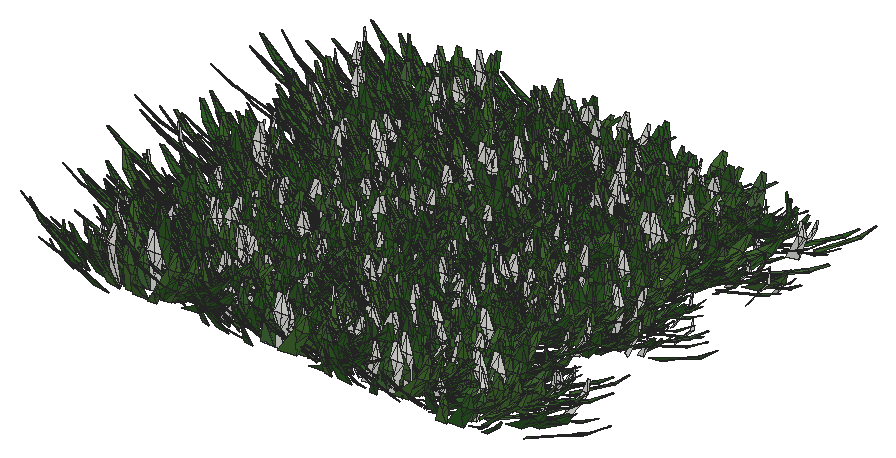
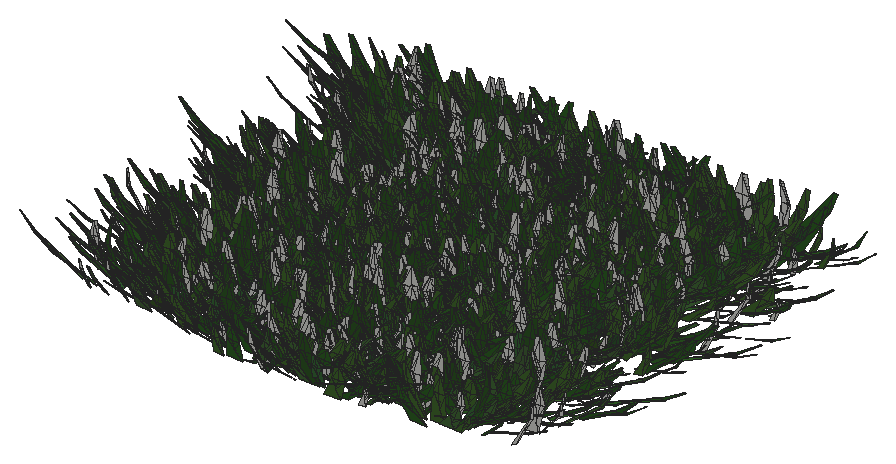
# SketchUp Ruby script. Lengths in inches.
U = 1.inch
M = Sketchup.active_model
def pt(a) = Geom::Point3d.new(a.map { |v| v * U })
def face(e, loops, mat)
  f = e.add_face(loops[0].map { |a| pt(a) })
  loops[1..].each { |l| e.add_face(l.map { |a| pt(a) }).erase! }
  f.material = f.back_material = mat if mat
  f
end
# faces: each face lists its corners as indices into pts; further lists are holes
def faces(e, pts, list, mat = nil) = list.each { |f| face(e, (f[0].is_a?(Array) ? f : [f]).map { |l| l.map { |i| pts[i] } }, mat) }
# xy, xz, yz: faces in a plane at the given z, y or x. An outline is a flat list of corners, or four numbers for a rectangle; further outlines are holes
def ring(l) = l.size == 4 ? [[l[0], l[1]], [l[2], l[1]], [l[2], l[3]], [l[0], l[3]]] : l.each_slice(2).to_a
def flat(e, list, mat, &to3) = list.each { |f| face(e, (f[0].is_a?(Array) ? f : [f]).map { |l| ring(l).map { |u, v| to3.(u, v) } }, mat) }
def xy(e, z, list, mat = nil) = flat(e, list, mat) { |x, y| [x, y, z] }
def xz(e, y, list, mat = nil) = flat(e, list, mat) { |x, z| [x, y, z] }
def yz(e, x, list, mat = nil) = flat(e, list, mat) { |y, z| [x, y, z] }
def lines(e, pts, list) = list.each { |a, b| e.add_line(pt(pts[a]), pt(pts[b])) }
# prism: a flat outline (further loops are holes) pulled along v
def prism(e, loops, v, mat = nil)
  f = face(e, loops, mat); d = Geom::Vector3d.new(v.map { |x| x * U })
  f.pushpull(f.normal.samedirection?(d) ? d.length : -d.length)
end
def box(e, o, s, mat = nil) = prism(e, [[o, [o[0] + s[0], o[1], o[2]], [o[0] + s[0], o[1] + s[1], o[2]], [o[0], o[1] + s[1], o[2]]]], [0, 0, s[2]], mat)
def at(x, y, z, deg = 0) = Geom::Transformation.translation(pt([x, y, z])) * Geom::Transformation.rotation(ORIGIN, Z_AXIS, deg.degrees)
def axes(o, x, y, z) = Geom::Transformation.new([*x, 0, *y, 0, *z, 0, *pt(o).to_a, 1])
def part(name) = M.definitions.add(name)
# library, detail: a bought-in or finely detailed component or shape, given as its bounding box
def library(name, o, s) = part(name).tap { |d| box(d.entities, o, s) }
def detail(e, o, s) = box(e.add_group.entities, o, s)
def put(e, d, t, mat = nil) = e.add_instance(d, t).tap { |i| i.material = mat if mat }
def group(e, t, mat = nil) = e.add_group.tap { |g| g.transformation = t; g.material = mat if mat }.entities
root = M.entities
M.materials.add("Material10").color = [48, 100, 38]
M.materials.add("Material3").color = [68, 110, 58]
M.materials.add("Material4").color = [48, 90, 38]
M.materials.add("Material5").color = [68, 110, 48]
M.materials.add("Material6").color = [48, 90, 48]
M.materials.add("Material7").color = [58, 110, 58]
M.materials.add("Material8").color = [58, 90, 38]
M.materials.add("Material9").color = [68, 100, 58]
c1 = part("grass00")
p = [[-0.6875,0.15,0],[-0.56,0.08,5.52],[-0.04,0.03,2.76],[0.48,-0.02,0],[0.35,-0.02,5.52],[-0.1,-0.14,5.52],
  [-0.12,0.65,8.37],[-0.42,0.65,8.37]]
faces(c1.entities,p,[[0,1,2,3],[3,2,4],[1,5,2],[5,4,2],[1,6,5],[4,5,6],[7,6,1]])
c2 = part("Group16\#1")
put(c2.entities,c1,axes([1.44,-0.61,-0.01],[0.05352,0.12609,0],[-0.10704,0.04543,0.07239],[0.06664,-0.02828,0.11628]),"Material6")
put(c2.entities,c1,axes([0.76,-0.15,-0.01],[0.04676,0.24062,0],[-0.23162,0.04501,0.06642],[0.0652,-0.01267,0.23595]),"Material3")
put(c2.entities,c1,axes([0.79,0.01,-0.01],[-0.00606,0.34651,0],[-0.34381,-0.00602,0.0432],[0.04319,0.00076,0.34386]))
put(c2.entities,c1,axes([1,0.23,-0.01],[-0.07192,0.31144,0],[-0.28722,-0.06632,0.1236],[0.12043,0.02781,0.29478]),"Material5")
put(c2.entities,c1,axes([1.66,0.77,-0.01],[-0.13828,0.29651,0],[-0.21551,-0.1005,0.22471],[0.20365,0.09498,0.23779]),"Material10")
put(c2.entities,c1,axes([0.6875,0.52,-0.01],[-0.18126,0.24051,0],[-0.22746,-0.17142,0.09788],[0.07817,0.05891,0.28481]),"Material5")
put(c2.entities,c1,axes([0.68,0.78,-0.01],[-0.215,0.18688,0],[-0.12385,-0.14248,0.21334],[0.13995,0.16101,0.18878]),"Material3")
put(c2.entities,c1,axes([0.56,1,-0.01],[-0.13756,0.07624,0],[-0.06159,-0.11112,0.0927],[0.04494,0.08108,0.12705]),"Material5")
put(c2.entities,c1,axes([0.2,0.64,-0.01],[-0.23729,0.07254,0],[-0.05711,-0.18681,0.153],[0.04473,0.14632,0.19535]),"Material10")
put(c2.entities,c1,axes([0.0625,0.72,-0.01],[-0.28874,0.02525,0],[-0.02179,-0.24916,0.14647],[0.01276,0.14591,0.25012]),"Material3")
put(c2.entities,c1,axes([-0.08,0.62,-0.01],[-0.34089,-0.04187,0],[0.03255,-0.26504,0.216],[-0.02633,0.21439,0.26703]),"Material10")
put(c2.entities,c1,axes([-0.34,0.98,-0.01],[-0.14314,-0.0493,0],[0.04397,-0.12769,0.06843],[-0.02228,0.0647,0.13505]),"Material10")
put(c2.entities,c1,axes([-0.87,1.45,-0.01],[-0.23488,-0.14114,0],[0.13761,-0.22901,0.06087],[-0.03135,0.05217,0.26717]))
put(c2.entities,c1,axes([-0.72,0.77,-0.01],[-0.14208,-0.13251,0],[0.07209,-0.0773,0.16301],[-0.11118,0.11922,0.1057]),"Material10")
put(c2.entities,c1,axes([-0.62,0.43,-0.01],[-0.14845,-0.21203,0],[0.18654,-0.13061,0.12304],[-0.10079,0.07057,0.22772]),"Material3")
put(c2.entities,c1,axes([-0.68,0.29,-0.01],[-0.13639,-0.32136,0],[0.31723,-0.13464,0.05579],[-0.05136,0.0218,0.34462]),"Material4")
put(c2.entities,c1,axes([-0.64,0.125,-0.01],[-0.0458,-0.23569,0],[0.22124,-0.043,0.08276],[-0.08124,0.01579,0.22538]),"Material7")
put(c2.entities,c1,axes([-1.6,-0.03,-0.01],[0.00576,-0.32897,0],[0.27526,0.00482,0.18018],[-0.18015,-0.00315,0.2753]),"Material5")
put(c2.entities,c1,axes([-1.36,-0.31,-0.01],[0.05718,-0.24765,0],[0.18172,0.04196,0.17267],[-0.16825,-0.03885,0.1865]),"Material10")
put(c2.entities,c1,axes([-1.54,-0.72,-0.01],[0.06537,-0.14017,0],[0.13555,0.06321,0.03939],[-0.0357,-0.01665,0.14956]))
put(c2.entities,c1,axes([-1.19,-0.9,-0.01],[0.09597,-0.12735,0],[0.11214,0.08451,0.07557],[-0.06035,-0.04548,0.14042]),"Material9")
put(c2.entities,c1,axes([-0.47,-0.54,-0.01],[0.11588,-0.10072,0],[0.0618,0.0711,0.12124],[-0.07953,-0.0915,0.0942]))
put(c2.entities,c1,axes([-0.47,-0.84,-0.01],[0.11927,-0.0661,0],[0.06603,0.11913,0.00646],[-0.00313,-0.00565,0.13621]),"Material5")
put(c2.entities,c1,axes([-0.38,-1.24,-0.01],[0.28037,-0.08571,0],[0.0618,0.20215,0.20315],[-0.05939,-0.19428,0.21139]),"Material9")
put(c2.entities,c1,axes([-0.06,-0.66,-0.01],[0.22719,-0.01987,0],[0.01247,0.14255,0.17758],[-0.01547,-0.17691,0.1431]),"Material8")
put(c2.entities,c1,axes([0.11,-0.89,-0.01],[0.14882,0.01828,0],[-0.01058,0.08611,0.12229],[0.01491,-0.12138,0.08676]),"Material6")
put(c2.entities,c1,axes([0.25,-0.72,-0.01],[0.20481,0.07053,0],[-0.06206,0.18022,0.10291],[0.03351,-0.0973,0.1906]),"Material6")
put(c2.entities,c1,axes([0.85,-1.42,-0.01],[0.16481,0.09904,0],[-0.09472,0.15762,0.05616],[0.02893,-0.04814,0.18389]),"Material5")
put(c2.entities,c1,axes([1.01,-1.09,-0.01],[0.21858,0.20385,0],[-0.17495,0.1876,0.15339],[0.10462,-0.11218,0.25652]),"Material10")
put(c2.entities,c1,axes([1.01,-0.71,-0.01],[0.08733,0.12473,0],[-0.06445,0.04512,0.13037],[0.1068,-0.07477,0.07867]),"Material6")
c3 = part("Group15\#1")
put(c3.entities,c2,at(0,0,0))
c4 = part("3darcstudiotree_grass00\#1")
put(c4.entities,c3,at(0,0,0))
put(root,c4,axes([922.19,902.96,0],[3.02119,-0.73797,0],[3.34783,0.85662,-0.03867],[0.15719,0.04022,1.7417]))
put(root,c4,axes([921.78,912.33,0],[-0.66076,1.04694,0],[-4.20152,-0.16573,-0.0149],[-0.10633,-0.00419,1.9212]))
put(root,c4,axes([924.36,916.55,0],[-4.31344,-0.70765,0],[2.03692,-0.77599,-0.04657],[0.20265,-0.0772,1.84036]))
put(root,c4,axes([924.04,895.31,0],[1.44261,-1.06055,0],[4.32057,0.36732,-0.01889],[0.12331,0.01048,1.96679]))
put(root,c4,axes([923.94,921.2,0],[2.7969,-0.77222,0],[3.1053,0.70294,-0.04299],[0.19432,0.04399,1.59659]))
put(root,c4,axes([924.92,894.38,0],[-3.32225,-0.97797,0],[3.38352,-0.71838,-0.05304],[0.28473,-0.06045,1.95407]))
put(root,c4,axes([924.86,922.86,0],[-4.68241,-0.00671,0],[0.02158,-0.94079,-0.00073],[0.00003,-0.00117,1.50826]))
put(root,c4,axes([924.16,924.21,0],[-2.30847,0.97502,0],[-3.8485,-0.56948,-0.03668],[-0.22363,-0.03309,1.98009]))
put(root,c4,axes([924.59,907.05,0],[-3.40463,0.90031,0],[-2.90136,-0.68574,-0.02847],[-0.11642,-0.02752,1.40417]))
put(root,c4,axes([925.07,925.48,0],[-3.76475,0.39529,0],[-1.59865,-0.95161,-0.01995],[-0.04859,-0.02892,1.62326]))
put(root,c4,axes([924.7,900.36,0],[-2.71864,0.85934,0],[-2.93369,-0.58007,-0.01059],[-0.0476,-0.00941,1.33934]))
put(root,c4,axes([925.75,913.93,0],[-4.9722,0.10596,0],[-0.33395,-0.9794,-0.04632],[-0.03038,-0.08909,1.89764]))
put(root,c4,axes([924,927.71,0],[3.97374,0.24333,0],[-1.22585,1.25118,-0.01455],[-0.02127,0.02171,1.97892]))
put(root,c4,axes([926.76,914.61,0],[-4.53093,-0.46907,0],[1.45069,-0.87579,-0.00358],[0.00956,-0.00577,1.65637]))
put(root,c4,axes([925.76,919.37,0],[-1.34638,0.95238,0],[-3.42274,-0.30242,-0.03966],[-0.22852,-0.02019,1.38647]))
put(root,c4,axes([926.29,911.04,0],[-3.83366,0.85497,0],[-2.76672,-0.77537,-0.04505],[-0.16078,-0.04506,1.39266]))
put(root,c4,axes([927.32,917.65,0],[-1.48823,-0.96446,0],[4.19205,-0.40429,-0.03571],[0.22835,-0.02202,1.92492]))
put(root,c4,axes([925.79,931.9375,0],[2.1454,0.98431,0],[-3.66531,0.49931,-0.025],[-0.16769,0.02284,1.99255]))
put(root,c4,axes([927.59,912.1,0],[-4.49935,0.03553,0],[-0.13779,-1.09065,-0.03959],[-0.00757,-0.05991,1.65212]))
put(root,c4,axes([926.65,904.93,0],[3.94822,-0.31947,0],[1.46453,1.13124,-0.01611],[0.0264,0.02039,1.58139]))
put(root,c4,axes([925.95,905.5,0],[3.048,0.98317,0],[-3.94868,0.7651,-0.03267],[-0.16044,0.03109,1.93988]))
put(root,c4,axes([926.13,929.33,0],[1.55836,1.05765,0],[-4.59334,0.423,-0.04046],[-0.19369,0.01784,1.56076]))
put(root,c4,axes([926.24,902.52,0],[0.02941,0.96921,0],[-5.11425,0.0097,-0.03677],[-0.15931,0.0003,1.38481]))
put(root,c4,axes([928.14,896.83,0],[-4.27197,-0.09913,0],[0.4691,-1.26352,-0.06502],[0.02705,-0.07286,1.42798]))
put(root,c4,axes([927.1,908.91,0],[-0.64236,0.88776,0],[-3.75703,-0.1699,-0.01415],[-0.08369,-0.00378,1.43376]))
put(root,c4,axes([928.22,901.49,0],[1.50582,-1.13859,0],[4.62077,0.38195,-0.04027],[0.21526,0.01779,1.71232]))
put(root,c4,axes([928.3125,930,0],[3.80605,-0.38984,0],[1.42887,0.87189,-0.00746],[0.01834,0.01119,1.52751]))
put(root,c4,axes([927.69,898.05,0],[3.10025,0.78829,0],[-3.57532,0.87883,-0.00938],[-0.04176,0.01026,1.95578]))
put(root,c4,axes([930.625,910.42,0],[-1.03913,-0.96879,0],[4.9712,-0.33326,-0.04199],[0.22449,-0.01505,1.7807]))
put(root,c4,axes([931.02,914.85,0],[-2.80799,-0.72862,0],[3.20036,-0.77086,-0.03217],[0.13224,-0.03185,1.58546]))
put(root,c4,axes([930.6875,901.37,0],[-4.63896,0.21302,0],[-0.93332,-1.27031,-0.05609],[-0.06093,-0.08294,1.94158]))
put(root,c4,axes([930.97,908.14,0],[-4.20413,-0.53147,0],[1.63067,-0.8062,-0.0255],[0.09899,-0.04894,1.94297]))
put(root,c4,axes([930.6,927.73,0],[-3.90893,0.68034,0],[-2.78299,-0.99937,-0.02528],[-0.08388,-0.03012,1.76765]))
put(root,c4,axes([930.33,898.82,0],[0.1527,1.05059,0],[-3.86386,0.0351,-0.04285],[-0.32383,0.00294,1.82733]))
put(root,c4,axes([930.53,926.14,0],[3.71157,-0.27079,0],[1.39023,1.19096,-0.04654],[0.05647,0.04838,1.34343]))
put(root,c4,axes([930.24,931.74,0],[3.97715,0.44667,0],[-1.63668,0.9108,-0.04301],[-0.1186,0.066,1.6797]))
put(root,c4,axes([930.86,908.72,0],[3.86502,-0.35215,0],[1.63703,1.12296,-0.06136],[0.12705,0.08716,1.80687]))
put(root,c4,axes([932.39,900.08,0],[-0.56967,-1.02254,0],[3.9547,-0.1377,-0.01078],[0.07697,-0.00268,1.79898]))
put(root,c4,axes([932.79,916.45,0],[-1.46525,-0.90866,0],[3.94836,-0.39793,-0.00075],[0.00398,-0.0004,1.52674]))
put(root,c4,axes([931.21,903.43,0],[4.11417,0.05124,0],[-0.24086,1.20875,-0.00527],[-0.00138,0.00693,1.59512]))
put(root,c4,axes([933.53,930.17,0],[-2.16831,-1.16182,0],[4.23849,-0.49439,-0.01753],[0.08143,-0.0095,1.49864]))
put(root,c4,axes([932.22,921.73,0],[3.83036,-0.81769,0],[2.5645,0.75081,-0.01134],[0.04499,0.01317,1.5074]))
put(root,c4,axes([933.03,897.48,0],[-4.70771,0.35936,0],[-1.47237,-1.20555,-0.03433],[-0.04305,-0.03525,1.35329]))
put(root,c4,axes([932.8,917.68,0],[-3.29867,0.81125,0],[-2.71253,-0.68934,-0.0233],[-0.12397,-0.0315,1.83382]))
put(root,c4,axes([932.52,919.77,0],[-0.78138,1.08578,0],[-4.54266,-0.20432,-0.02584],[-0.11477,-0.00516,1.30174]))
put(root,c4,axes([933.79,923.92,0],[2.17808,-0.78505,0],[4.26827,0.74013,-0.02169],[0.08641,0.01498,1.57389]))
put(root,c4,axes([932.86,904.5,0],[-0.70651,0.89155,0],[-4.48869,-0.22232,-0.03573],[-0.20534,-0.01017,1.67549]))
put(root,c4,axes([934.39,895.2,0],[-3.74457,-0.22418,0],[0.88563,-0.92456,-0.00326],[0.00619,-0.00646,1.93944]))
put(root,c4,axes([932.75,906.34,0],[3.07381,0.68375,0],[-2.58138,0.72529,-0.00943],[-0.03598,0.01011,1.39243]))
put(root,c4,axes([933.5625,911.76,0],[-0.98652,1.16576,0],[-4.8711,-0.25764,-0.05558],[-0.27807,-0.01471,1.59125]))
put(root,c4,axes([934.34,928.53,0],[1.84217,-1.02173,0],[3.32278,0.37443,-0.02223],[0.14494,0.01633,1.62899]))
put(root,c4,axes([934.43,922.28,0],[3.84212,-0.38705,0],[1.37613,0.85378,-0.02314],[0.05053,0.03135,1.34449]))
put(root,c4,axes([933.86,913.49,0],[1.9287,1.10406,0],[-3.72338,0.40653,-0.01938],[-0.11115,0.01214,1.58937]))
put(root,c4,axes([936.25,907.91,0],[-1.7561,-0.89869,0],[3.62331,-0.44251,-0.0349],[0.22933,-0.02801,1.84302]))
put(root,c4,axes([936.89,917.16,0],[-4.2283,-0.0064,0],[0.03055,-1.26138,-0.0591],[0.00173,-0.07136,1.52309]))
put(root,c4,axes([937.11,914.2,0],[-4.7095,-0.098,0],[0.36806,-1.10545,-0.036],[0.02101,-0.06311,1.9513]))
put(root,c4,axes([936.86,925.27,0],[1.82992,-1.20621,0],[3.40004,0.32238,-0.00605],[0.04862,0.00461,1.95327]))
put(root,c4,axes([936.97,933.53,0],[1.45443,-0.84507,0],[4.00274,0.43056,-0.02985],[0.15547,0.01672,1.54439]))
put(root,c4,axes([936.65,922.17,0],[0.91767,-0.96683,0],[3.51247,0.20837,-0.04624],[0.38905,0.02308,1.95114]))
put(root,c4,axes([936.64,928.94,0],[-2.22547,0.97496,0],[-3.23871,-0.46204,-0.04437],[-0.2422,-0.03455,1.46464]))
put(root,c4,axes([936.25,899.97,0],[-1.07117,1.0548,0],[-4.16401,-0.26429,-0.01715],[-0.09038,-0.00574,1.46021]))
put(root,c4,axes([937.97,918,0],[-0.7412,-1.17343,0],[4.56586,-0.18025,-0.01303],[0.08774,-0.00346,1.96953]))
put(root,c4,axes([937.62,894.28,0],[1.34034,-1.07316,0],[4.75764,0.37138,-0.04262],[0.23721,0.01852,1.81655]))
put(root,c4,axes([938.28,910.15,0],[-4.70029,0.25343,0],[-0.93391,-1.08255,-0.00845],[-0.00874,-0.01013,1.35873]))
put(root,c4,axes([937.6875,903.02,0],[-2.69017,1.10468,0],[-3.43594,-0.52296,-0.03488],[-0.16243,-0.02472,1.37068]))
put(root,c4,axes([937.2,906.39,0],[3.70476,-0.12271,0],[0.5167,0.975,-0.04905],[0.03883,0.07327,1.48186]))
put(root,c4,axes([937.92,912.17,0],[-3.18848,0.90294,0],[-3.14265,-0.69359,-0.01581],[-0.06022,-0.01329,1.33135]))
put(root,c4,axes([937.88,897.4375,0],[3.51285,-0.33152,0],[1.41112,0.93454,-0.04981],[0.11878,0.07867,1.68613]))
put(root,c4,axes([939.23,897.92,0],[-0.91328,-1.0252,0],[3.54973,-0.19764,-0.00779],[0.04648,-0.00259,1.38852]))
put(root,c4,axes([939.26,915.54,0],[-2.2581,-1.00308,0],[3.75758,-0.52868,-0.05229],[0.27859,-0.0392,1.64764]))
put(root,c4,axes([939.36,904.59,0],[0.44969,-0.9198,0],[4.71868,0.14419,-0.02785],[0.1393,0.00426,1.49696]))
put(root,c4,axes([938.37,909.17,0],[-2.40206,1.15116,0],[-4.41351,-0.57559,-0.04188],[-0.22518,-0.02937,1.88687]))
put(root,c4,axes([937.69,924.38,0],[3.15973,0.64464,0],[-2.80076,0.858,-0.03119],[-0.13565,0.04156,1.90467]))
put(root,c4,axes([938.93,931.97,0],[-2.00451,1.10371,0],[-3.34752,-0.37998,-0.0444],[-0.28643,-0.03251,1.62807]))
put(root,c4,axes([939.31,919.32,0],[-2.48346,0.94681,0],[-4.13972,-0.67865,-0.05216],[-0.1846,-0.03026,1.30947]))
put(root,c4,axes([939.3,920.8,0],[-2.01885,1.11907,0],[-4.67604,-0.52724,-0.03185],[-0.16487,-0.01859,1.82087]))
put(root,c4,axes([939.4,901.55,0],[2.27461,0.70298,0],[-2.88603,0.58364,-0.02717],[-0.1658,0.03353,1.82093]))
put(root,c4,axes([939.51,895.42,0],[3.78924,0.26456,0],[-0.97261,0.87066,-0.03829],[-0.06398,0.05727,1.40372]))
put(root,c4,axes([940.08,927.6,0],[4.35332,-0.20638,0],[0.96031,1.26603,-0.05959],[0.0538,0.07093,1.56123]))
put(root,c4,axes([940.22,929.95,0],[0.89231,1.23104,0],[-4.86402,0.22035,-0.02342],[-0.12734,0.00577,1.70718]))
put(root,c4,axes([942.52,895.18,0],[-3.95423,-0.27375,0],[1.31501,-1.1872,-0.02644],[0.04369,-0.03944,1.9068]))
put(root,c4,axes([943.3,922.88,0],[-4.2551,-0.55246,0],[2.21747,-1.06745,-0.03725],[0.08878,-0.04274,1.55507]))
put(root,c4,axes([942.43,931.7,0],[-2.9637,1.00971,0],[-3.98182,-0.73047,-0.06171],[-0.27775,-0.05095,1.72322]))
put(root,c4,axes([942.15,926.875,0],[1.86969,0.78057,0],[-3.16238,0.47343,-0.04808],[-0.33365,0.04995,1.86326]))
put(root,c4,axes([942.11,914.82,0],[4.806,-0.14737,0],[0.47152,0.96109,-0.03723],[0.02452,0.04998,1.30959]))
put(root,c4,axes([943.58,928.62,0],[0.365,-1.172,0],[4.21149,0.08198,-0.01871],[0.12678,0.00247,1.79426]))
put(root,c4,axes([944.16,916.93,0],[-2.38517,-0.85712,0],[3.89197,-0.67691,-0.03629],[0.14533,-0.02528,1.44541]))
put(root,c4,axes([944.26,913.53,0],[-2.55212,-0.67388,0],[3.75826,-0.88958,-0.06171],[0.2261,-0.05352,1.63202]))
put(root,c4,axes([944.47,898.12,0],[0.94935,-1.13668,0],[4.79838,0.25048,-0.01659],[0.08229,0.0043,1.55232]))
put(root,c4,axes([945.08,924.8,0],[-4.47557,-0.42377,0],[1.78381,-1.17745,-0.00084],[0.00126,-0.00083,1.34285]))
put(root,c4,axes([944.21,921.34,0],[-2.98855,0.54778,0],[-2.22427,-0.75844,-0.03589],[-0.17423,-0.05941,1.93035]))
put(root,c4,axes([943.62,920.11,0],[3.78365,-0.18577,0],[0.80923,1.03012,-0.00241],[0.00316,0.00403,1.79003]))
put(root,c4,axes([944.16,918.55,0],[-1.65227,1.03376,0],[-3.9595,-0.39553,-0.0529],[-0.2919,-0.02916,1.58349]))
put(root,c4,axes([943.6,905.69,0],[1.52496,0.98405,0],[-3.48981,0.338,-0.02409],[-0.15435,0.01495,1.60735]))
put(root,c4,axes([943.48,897.12,0],[5.01381,0.29286,0],[-0.86637,0.92702,-0.04207],[-0.05348,0.05723,1.32997]))
put(root,c4,axes([944.84,902.66,0],[-3.05375,0.95057,0],[-3.1621,-0.6349,-0.04358],[-0.22353,-0.04488,1.66757]))
put(root,c4,axes([944.08,911.96,0],[3.93232,0.3892,0],[-1.53002,0.96616,-0.03237],[-0.07493,0.04731,1.63378]))
put(root,c4,axes([945.3,933.13,0],[-3.88658,0.80784,0],[-2.79245,-0.83967,-0.00935],[-0.03544,-0.01066,1.61847]))
put(root,c4,axes([945.09,910.16,0],[3.7138,-0.79833,0],[2.34942,0.68309,-0.0226],[0.10849,0.03154,1.65792]))
put(root,c4,axes([946.33,926.19,0],[-4.61826,-0.0324,0],[0.10564,-0.94117,-0.03959],[0.00926,-0.08249,1.96257]))
put(root,c4,axes([944.65,909.16,0],[4.49063,0.58178,0],[-2.32504,1.12165,-0.0509],[-0.11953,0.05767,1.61215]))
put(root,c4,axes([945.4,907.94,0],[4.04347,-0.18678,0],[0.90955,1.23062,-0.01263],[0.0127,0.01719,1.73191]))
put(root,c4,axes([946.15,901.66,0],[3.03325,-1.05553,0],[3.12611,0.56147,-0.0087],[0.04718,0.00847,1.60603]))
put(root,c4,axes([946.41,904.55,0],[3.36364,-0.39705,0],[1.75914,0.93141,-0.03456],[0.09555,0.05059,1.66747]))
put(root,c4,axes([946.51,929.84,0],[-0.83011,0.88053,0],[-3.59902,-0.21206,-0.04738],[-0.28817,-0.01698,1.4441]))
put(root,c4,axes([945.76,900.47,0],[2.92685,0.95557,0],[-3.59966,0.68909,-0.02004],[-0.07664,0.01467,1.3651]))
put(root,c4,axes([948.7,919.82,0],[-3.8765,-0.37875,0],[1.47892,-0.94605,-0.02269],[0.05344,-0.03418,1.64292]))
put(root,c4,axes([948.48,901.3125,0],[-4.50586,0.35674,0],[-1.23927,-0.9783,-0.01419],[-0.02922,-0.02307,1.75006]))
put(root,c4,axes([948.28,894.08,0],[2.37725,-0.90712,0],[3.87375,0.63448,-0.04807],[0.23586,0.03863,1.69791]))
put(root,c4,axes([948.46,910.67,0],[2.75939,-0.81589,0],[3.35102,0.70833,-0.03628],[0.15055,0.03182,1.49031]))
put(root,c4,axes([949.34,925.45,0],[-1.86432,-1.00241,0],[3.34424,-0.38873,-0.04244],[0.31797,-0.03696,1.90455]))
put(root,c4,axes([949.36,895.375,0],[1.78946,-1.14425,0],[3.5583,0.3478,-0.00888],[0.06487,0.00634,1.87213]))
put(root,c4,axes([948.34,896.44,0],[-1.11444,1.02351,0],[-4.99646,-0.34002,-0.0223],[-0.10571,-0.00719,1.58974]))
put(root,c4,axes([950.12,930.57,0],[-1.04914,-1.06304,0],[3.77307,-0.23273,-0.01268],[0.08139,-0.00502,1.60602]))
put(root,c4,axes([950.62,911.77,0],[-2.07823,-1.0748,0],[4.05386,-0.48991,-0.04214],[0.21023,-0.02541,1.55921]))
put(root,c4,axes([949.82,926.84,0],[-3.28261,0.64166,0],[-2.52163,-0.80626,-0.02144],[-0.10036,-0.03209,1.94421]))
put(root,c4,axes([949.1875,916.54,0],[-0.6945,0.99441,0],[-4.06846,-0.17759,-0.03794],[-0.20649,-0.00901,1.42617]))
put(root,c4,axes([949.8,899.62,0],[-2.06095,0.96891,0],[-3.40314,-0.45242,-0.04799],[-0.3505,-0.0466,1.99284]))
put(root,c4,axes([950.94,906.42,0],[-2.17627,-1.09913,0],[3.44474,-0.42628,-0.01272],[0.06522,-0.00807,1.37453]))
put(root,c4,axes([950.6875,931.5625,0],[0.22128,-1.19645,0],[4.67967,0.05409,-0.04434],[0.23423,0.00271,1.54852]))
put(root,c4,axes([951.64,907.74,0],[-3.09718,-0.64135,0],[2.64207,-0.79743,-0.01497],[0.06729,-0.02031,1.82381]))
put(root,c4,axes([950.0625,897.98,0],[-1.82154,1.01586,0],[-4.52061,-0.50662,-0.00369],[-0.01716,-0.00192,1.57624]))
put(root,c4,axes([950.87,904.79,0],[-3.65354,0.89474,0],[-2.56614,-0.6549,-0.00183],[-0.00785,-0.002,1.40539]))
put(root,c4,axes([950.67,921.35,0],[-2.50195,1.12274,0],[-4.19712,-0.58456,-0.0557],[-0.2512,-0.03499,1.55009]))
put(root,c4,axes([952.07,923.96,0],[-3.5144,-0.95148,0],[3.77994,-0.8726,-0.04946],[0.16772,-0.03872,1.48426]))
put(root,c4,axes([951.86,914.69,0],[-4.39725,-0.1693,0],[0.59529,-0.96636,-0.03709],[0.03896,-0.06324,1.68681]))
put(root,c4,axes([951.49,913.5,0],[-3.41733,0.39454,0],[-1.99566,-1.08035,-0.05064],[-0.10494,-0.05681,1.47033]))
put(root,c4,axes([952.31,903.15,0],[0.92698,-1.20285,0],[4.36209,0.2101,-0.00212],[0.01245,0.0006,1.6588]))
put(root,c4,axes([951.66,928.74,0],[3.47512,-0.34723,0],[1.8254,1.14182,-0.02256],[0.04248,0.02657,1.55958]))
put(root,c4,axes([952.2,922.21,0],[2.15551,-0.74125,0],[3.38784,0.61573,-0.02782],[0.16259,0.02955,1.89124]))
put(root,c4,axes([951.62,909.47,0],[2.61248,0.6584,0],[-3.28353,0.8143,-0.03885],[-0.15165,0.03761,1.58937]))
put(root,c4,axes([952.22,918.65,0],[3.40608,0.31789,0],[-1.62863,1.09064,-0.03179],[-0.06759,0.04526,1.76952]))
put(root,c4,axes([954.31,915.4,0],[-1.7547,-0.95302,0],[3.61048,-0.41547,-0.04546],[0.29745,-0.03423,1.78943]))
put(root,c4,axes([954.7,916.87,0],[1.053,-0.96727,0],[3.62694,0.24678,-0.01758],[0.12396,0.00843,1.71636]))
put(root,c4,axes([955.11,901.57,0],[-3.98559,-0.40727,0],[1.42948,-0.87432,-0.04864],[0.11159,-0.06825,1.4319]))
put(root,c4,axes([955.24,922.1875,0],[-1.88311,-0.95255,0],[4.51474,-0.55783,-0.04891],[0.26234,-0.03241,1.88309]))
put(root,c4,axes([955.51,931.5,0],[-4.25078,-0.391,0],[1.69928,-1.15461,-0.01333],[0.0258,-0.01753,1.7245]))
put(root,c4,axes([955.04,899.93,0],[-0.58963,-1.12221,0],[3.81516,-0.12529,-0.04534],[0.30342,-0.00996,1.62314]))
put(root,c4,axes([955.46,909.05,0],[0.02643,-0.92207,0],[3.81186,0.00683,-0.01704],[0.12849,0.00023,1.79616]))
put(root,c4,axes([954.17,929.91,0],[-1.16899,0.9922,0],[-4.24579,-0.31264,-0.01201],[-0.06083,-0.00448,1.46096]))
put(root,c4,axes([955.9,913.11,0],[-1.37406,-1.03466,0],[4.06189,-0.33714,-0.03393],[0.15904,-0.0132,1.3212]))
put(root,c4,axes([954.69,894.09,0],[4.45768,-0.32922,0],[1.38468,1.17179,-0.05518],[0.09073,0.07678,1.77288]))
put(root,c4,axes([956.42,897.03,0],[1.09423,-1.18623,0],[4.14621,0.23904,-0.00305],[0.01978,0.00114,1.76865]))
put(root,c4,axes([955.53,910.98,0],[-2.60907,0.74079,0],[-3.52374,-0.77567,-0.02335],[-0.09985,-0.02198,1.67208]))
put(root,c4,axes([954.79,924.36,0],[0.14823,0.94449,0],[-4.53661,0.0445,-0.00595],[-0.04152,0.00041,1.98232]))
put(root,c4,axes([956.01,925.6,0],[-3.76988,0.83286,0],[-3.11368,-0.88087,-0.04086],[-0.13444,-0.03803,1.46035]))
put(root,c4,axes([956.27,911.73,0],[2.7445,-0.91806,0],[3.21973,0.60158,-0.03861],[0.21673,0.04049,1.76068]))
put(root,c4,axes([957.1,897.95,0],[0.91501,-1.15723,0],[4.8883,0.24157,-0.04547],[0.24719,0.01222,1.72572]))
